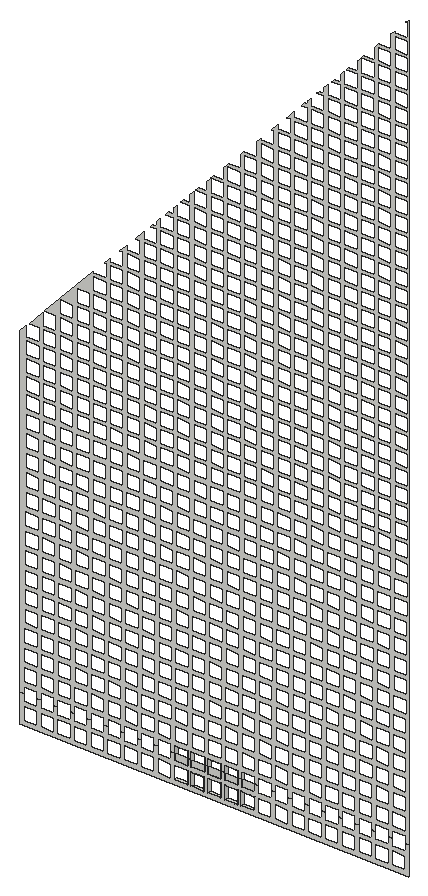
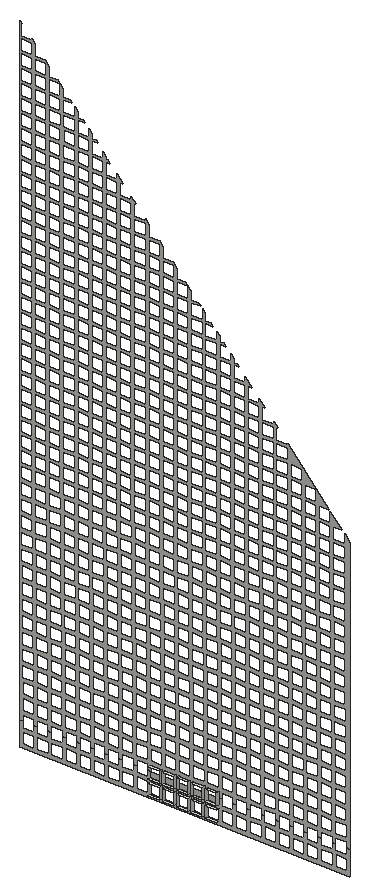
# SketchUp Ruby script. Lengths in inches.
U = 1.inch
M = Sketchup.active_model
def pt(a) = Geom::Point3d.new(a.map { |v| v * U })
def face(e, loops, mat)
  f = e.add_face(loops[0].map { |a| pt(a) })
  loops[1..].each { |l| e.add_face(l.map { |a| pt(a) }).erase! }
  f.material = f.back_material = mat if mat
  f
end
# faces: each face lists its corners as indices into pts; further lists are holes
def faces(e, pts, list, mat = nil) = list.each { |f| face(e, (f[0].is_a?(Array) ? f : [f]).map { |l| l.map { |i| pts[i] } }, mat) }
# xy, xz, yz: faces in a plane at the given z, y or x. An outline is a flat list of corners, or four numbers for a rectangle; further outlines are holes
def ring(l) = l.size == 4 ? [[l[0], l[1]], [l[2], l[1]], [l[2], l[3]], [l[0], l[3]]] : l.each_slice(2).to_a
def flat(e, list, mat, &to3) = list.each { |f| face(e, (f[0].is_a?(Array) ? f : [f]).map { |l| ring(l).map { |u, v| to3.(u, v) } }, mat) }
def xy(e, z, list, mat = nil) = flat(e, list, mat) { |x, y| [x, y, z] }
def xz(e, y, list, mat = nil) = flat(e, list, mat) { |x, z| [x, y, z] }
def yz(e, x, list, mat = nil) = flat(e, list, mat) { |y, z| [x, y, z] }
def lines(e, pts, list) = list.each { |a, b| e.add_line(pt(pts[a]), pt(pts[b])) }
# prism: a flat outline (further loops are holes) pulled along v
def prism(e, loops, v, mat = nil)
  f = face(e, loops, mat); d = Geom::Vector3d.new(v.map { |x| x * U })
  f.pushpull(f.normal.samedirection?(d) ? d.length : -d.length)
end
def box(e, o, s, mat = nil) = prism(e, [[o, [o[0] + s[0], o[1], o[2]], [o[0] + s[0], o[1] + s[1], o[2]], [o[0], o[1] + s[1], o[2]]]], [0, 0, s[2]], mat)
def at(x, y, z, deg = 0) = Geom::Transformation.translation(pt([x, y, z])) * Geom::Transformation.rotation(ORIGIN, Z_AXIS, deg.degrees)
def axes(o, x, y, z) = Geom::Transformation.new([*x, 0, *y, 0, *z, 0, *pt(o).to_a, 1])
def part(name) = M.definitions.add(name)
# library, detail: a bought-in or finely detailed component or shape, given as its bounding box
def library(name, o, s) = part(name).tap { |d| box(d.entities, o, s) }
def detail(e, o, s) = box(e.add_group.entities, o, s)
def put(e, d, t, mat = nil) = e.add_instance(d, t).tap { |i| i.material = mat if mat }
def group(e, t, mat = nil) = e.add_group.tap { |g| g.transformation = t; g.material = mat if mat }.entities
root = M.entities
xy(root,259.68,[[2231.87,480.14,2234.18,480.77],[2234.78,480.14,2237.09,480.77],[2237.69,480.14,2240.01,480.77],[2240.61,480.14,2242.92,480.77],[2243.52,480.14,2245.83,480.77]])
xy(root,262,[[2231.87,480.14,2234.18,480.77],[2234.78,480.14,2237.09,480.77],[2237.69,480.14,2240.01,480.77],[2240.61,480.14,2242.92,480.77],[2243.52,480.14,2245.83,480.77]])
xy(root,262.73,[[2231.9,480.14,2234.21,480.77],[2234.8125,480.14,2237.125,480.77],[2237.72,480.14,2240.04,480.77],[2240.64,480.14,2242.95,480.77],[2243.55,480.14,2245.86,480.77]])
xy(root,265.04,[[2231.9,480.14,2234.21,480.77],[2234.8125,480.14,2237.125,480.77],[2237.72,480.14,2240.04,480.77],[2240.64,480.14,2242.95,480.77],[2243.55,480.14,2245.86,480.77]])
xz(root,480.14,[[[2205.04,258.95,2272.64,258.95,2272.64,263.89,2272.07,263.89,2272.07,262.73,2269.76,262.73,2269.76,263.89,2269.16,263.89,2269.16,262.73,2266.84,262.73,2266.84,263.89,2266.24,263.89,2266.24,262.73,2263.93,262.73,2263.93,263.89,2263.33,263.89,2263.33,262.73,2261.02,262.73,2261.02,263.89,2260.42,263.89,2260.42,262.73,2258.11,262.73,2258.11,263.89,2257.51,263.89,2257.51,262.73,2255.2,262.73,2255.2,263.89,2254.6,263.89,2254.6,262.73,2252.28,262.73,2252.28,263.89,2251.68,263.89,2251.68,262.73,2249.37,262.73,2249.37,263.89,2248.77,263.89,2248.77,262.73,2246.46,262.73,2246.46,263.89,2245.86,263.89,2245.86,262.73,2243.55,262.73,2243.55,263.89,2242.95,263.89,2242.95,262.73,2240.64,262.73,2240.64,263.89,2240.04,263.89,2240.04,262.73,2237.72,262.73,2237.72,263.89,2237.125,263.89,2237.125,262.73,2234.8125,262.73,2234.8125,263.89,2234.21,263.89,2234.21,262.73,2231.9,262.73,2231.9,263.89,2231.3,263.89,2231.3,262.73,2228.99,262.73,2228.99,263.89,2228.39,263.89,2228.39,262.73,2226.08,262.73,2226.08,263.89,2225.48,263.89,2225.48,262.73,2223.16,262.73,2223.16,263.89,2222.5625,263.89,2222.5625,262.73,2220.25,262.73,2220.25,263.89,2219.65,263.89,2219.65,262.73,2217.34,262.73,2217.34,263.89,2216.74,263.89,2216.74,262.73,2214.43,262.73,2214.43,263.89,2213.83,263.89,2213.83,262.73,2211.52,262.73,2211.52,263.89,2210.92,263.89,2210.92,262.73,2208.6,262.73,2208.6,263.89,2208,263.89,2208,262.73,2205.69,262.73,2205.69,263.89,2205.04,263.89],[2269.73,259.68,2272.04,262],[2266.81,259.68,2269.13,262],[2263.9,259.68,2266.22,262],[2260.99,259.68,2263.3,262],[2258.08,259.68,2260.39,262],[2255.17,259.68,2257.48,262],[2252.25,259.68,2254.57,262],[2249.34,259.68,2251.66,262],[2246.43,259.68,2248.74,262],[2243.52,259.68,2245.83,262],[2240.61,259.68,2242.92,262],[2237.69,259.68,2240.01,262],[2234.78,259.68,2237.09,262],[2231.87,259.68,2234.18,262],[2228.96,259.68,2231.27,262],[2226.05,259.68,2228.36,262],[2223.13,259.68,2225.45,262],[2220.22,259.68,2222.53,262],[2217.31,259.68,2219.62,262],[2214.4,259.68,2216.71,262],[2211.49,259.68,2213.8,262],[2208.57,259.68,2210.89,262],[2205.66,259.68,2207.97,262]],[2231.9,262.73,2234.21,263.89],[2234.8125,262.73,2237.125,263.89],[2237.72,262.73,2240.04,263.89],[2240.64,262.73,2242.95,263.89],
  [2243.55,262.73,2245.86,263.89],[[2205.04,263.89,2205.69,263.89,2205.69,265.04,2208,265.04,2208,263.89,2208.6,263.89,2208.6,265.04,2210.92,265.04,2210.92,263.89,2211.52,263.89,2211.52,265.04,2213.83,265.04,2213.83,263.89,2214.43,263.89,2214.43,265.04,2216.74,265.04,2216.74,263.89,2217.34,263.89,2217.34,265.04,2219.65,265.04,2219.65,263.89,2220.25,263.89,2220.25,265.04,2222.5625,265.04,2222.5625,263.89,2223.16,263.89,2223.16,265.04,2225.48,265.04,2225.48,263.89,2226.08,263.89,2226.08,265.04,2228.39,265.04,2228.39,263.89,2228.99,263.89,2228.99,265.04,2231.3,265.04,2231.3,263.89,2231.9,263.89,2231.9,265.04,2234.21,265.04,2234.21,263.89,2234.8125,263.89,2234.8125,265.04,2237.125,265.04,2237.125,263.89,2237.72,263.89,2237.72,265.04,2240.04,265.04,2240.04,263.89,2240.64,263.89,2240.64,265.04,2242.95,265.04,2242.95,263.89,2243.55,263.89,2243.55,265.04,2245.86,265.04,2245.86,263.89,2246.46,263.89,2246.46,265.04,2248.77,265.04,2248.77,263.89,2249.37,263.89,2249.37,265.04,2251.68,265.04,2251.68,263.89,2252.28,263.89,2252.28,265.04,2254.6,265.04,2254.6,263.89,2255.2,263.89,2255.2,265.04,2257.51,265.04,2257.51,263.89,2258.11,263.89,2258.11,265.04,2260.42,265.04,2260.42,263.89,2261.02,263.89,2261.02,265.04,2263.33,265.04,2263.33,263.89,2263.93,263.89,2263.93,265.04,2266.24,265.04,2266.24,263.89,2266.84,263.89,2266.84,265.04,2269.16,265.04,2269.16,263.89,2269.76,263.89,2269.76,265.04,2272.07,265.04,2272.07,263.89,2272.64,263.89,2272.64,392.36,2272.21,391.9,2272.5,391.9,2272.5,389.59,2270.19,389.59,2270.19,389.75,2269.59,389.11,2269.59,386.84,2267.46,386.84,2266.68,386,2266.68,384.09,2264.89,384.09,2264.57,383.75,2264.48,383.65,2266.68,383.65,2266.68,381.34,2264.37,381.34,2264.37,383.53,2263.77,382.89,2263.77,381.34,2262.31,381.34,2261.9,380.9,2263.77,380.9,2263.77,378.59,2261.45,378.59,2261.45,380.43,2260.86,379.79,2260.86,378.59,2259.73,378.59,2259.32,378.15,2260.86,378.15,2260.86,375.84,2258.54,375.84,2258.54,377.32,2257.94,376.68,2257.94,375.84,2257.15,375.84,2256.74,375.4,2257.94,375.4,2257.94,373.09,2255.63,373.09,2255.63,374.21,2255.03,373.57,2255.03,373.09,2254.58,373.09,2254.11,372.59,2255.03,372.59,2255.03,370.27,2252.72,370.27,2252.72,371.11,2252.12,370.47,2252.12,370.27,2251.94,370.27,2251.47,369.77,2252.12,369.77,2252.12,367.46,2249.81,367.46,2249.81,368,2248.83,366.96,2249.21,366.96,2249.21,364.65,2246.89,364.65,2246.89,364.89,2246.2,364.15,2246.29,364.15,2246.29,361.84,2244.03,361.84,2243.38,361.14,2243.38,359.02,2241.4,359.02,2240.47,358.04,2240.47,356.21,2238.76,356.21,2238.29,355.71,2240.47,355.71,2240.47,353.4,2238.16,353.4,2238.16,355.57,2237.56,354.93,2237.56,353.4,2236.12,353.4,2235.65,352.9,2237.56,352.9,2237.56,350.59,2235.25,350.59,2235.25,352.46,2234.65,351.82,2234.65,350.59,2233.49,350.59,2233.02,350.09,2234.65,350.09,2234.65,347.77,2232.33,347.77,2232.33,349.36,2231.73,348.72,2231.73,347.77,2230.85,347.77,2230.38,347.27,2231.73,347.27,2231.73,344.96,2229.42,344.96,2229.42,346.25,2228.82,345.61,2228.82,344.96,2228.21,344.96,2227.75,344.46,2228.82,344.46,2228.82,342.15,2226.51,342.15,2226.51,343.14,2225.11,341.65,2225.91,341.65,2225.91,339.34,2223.6,339.34,2223.6,340.04,2222.47,338.84,2223,338.84,2223,336.52,2220.6875,336.52,2220.6875,336.93,2219.84,336.02,2220.09,336.02,2220.09,333.71,2217.77,333.71,2217.77,333.82,2209.29,324.77,2211.35,324.77,2211.35,322.46,2209.04,322.46,2209.04,324.5,2206.66,321.96,2208.4375,321.96,2208.4375,319.65,2206.125,319.65,2206.125,321.39,2205.04,320.24],[2270.19,375.84,2272.5,378.15],[2267.25,373.09,2269.57,375.4],[2270.19,373.09,2272.5,375.4],[2267.25,370.27,2269.57,372.59],[2270.19,370.27,2272.5,372.59],[2258.52,370.27,2260.83,372.59],[2261.45,370.27,2263.77,372.59],[2261.43,373.09,2263.74,375.4],[2264.37,373.09,2266.68,375.4],[2264.34,375.84,2266.65,378.15],[2267.28,375.84,2269.59,378.15],[2267.25,378.59,2269.57,380.9],[2270.19,378.59,2272.5,380.9],[2267.25,381.34,2269.57,383.65],[2270.19,381.34,2272.5,383.65],[2238.16,350.59,2240.47,352.9],[2235.25,347.77,2237.56,350.09],[2238.16,347.77,2240.47,350.09],[2232.33,344.96,2234.65,347.27],[2235.25,344.96,2237.56,347.27],[2238.16,344.96,2240.47,347.27],[2241.07,344.96,2243.38,347.27],[2243.98,344.96,2246.29,347.27],[2246.89,344.96,2249.21,347.27],[2249.81,344.96,2252.12,347.27],[2252.72,344.96,2255.03,347.27],[2255.63,344.96,2257.94,347.27],[2258.54,344.96,2260.86,347.27],[2261.45,344.96,2263.77,347.27],[2264.37,344.96,2266.68,347.27],[2267.28,344.96,2269.59,347.27],[2270.19,344.96,2272.5,347.27],[2241.07,347.77,2243.38,350.09],[2243.98,347.77,2246.29,350.09],[2246.89,347.77,2249.21,350.09],[2249.81,347.77,2252.12,350.09],[2252.72,347.77,2255.03,350.09],[2255.63,347.77,2257.94,350.09],[2258.54,347.77,2260.86,350.09],[2261.45,347.77,2263.77,350.09],[2264.37,347.77,2266.68,350.09],[2267.28,347.77,2269.59,350.09],[2270.19,347.77,2272.5,350.09],[2241.07,350.59,2243.38,352.9],[2243.98,350.59,2246.29,352.9],[2246.89,350.59,2249.21,352.9],[2249.81,350.59,2252.12,352.9],[2252.72,350.59,2255.03,352.9],[2255.63,350.59,2257.94,352.9],[2258.54,350.59,2260.86,352.9],[2261.45,350.59,2263.77,352.9],[2264.37,350.59,2266.68,352.9],[2267.28,350.59,2269.59,352.9],[2270.19,350.59,2272.5,352.9],[2241.07,353.4,2243.38,355.71],[2243.98,353.4,2246.29,355.71],[2246.89,353.4,2249.21,355.71],[2249.81,353.4,2252.12,355.71],[2252.72,353.4,2255.03,355.71],[2255.63,353.4,2257.94,355.71],[2258.54,353.4,2260.86,355.71],[2261.45,353.4,2263.77,355.71],[2264.37,353.4,2266.68,355.71],[2267.28,353.4,2269.59,355.71],[2270.19,353.4,2272.5,355.71],[2252.72,367.46,2255.03,369.77],[2255.63,367.46,2257.94,369.77],[2264.37,367.46,2266.68,369.77],[2270.19,367.46,2272.5,369.77],[2261.45,367.46,2263.77,369.77],[2258.54,367.46,2260.86,369.77],[2267.28,367.46,2269.59,369.77],[2252.72,364.65,2255.03,366.96],[2258.54,364.65,2260.86,366.96],[2267.28,364.65,2269.59,366.96],[2264.37,364.65,2266.68,366.96],[2255.63,364.65,2257.94,366.96],[2261.45,364.65,2263.77,366.96],[2270.19,364.65,2272.5,366.96],[2249.81,364.65,2252.12,366.96],[2261.45,361.84,2263.77,364.15],[2267.28,361.84,2269.59,364.15],[2255.63,361.84,2257.94,364.15],[2258.54,361.84,2260.86,364.15],[2270.19,361.84,2272.5,364.15],[2249.81,361.84,2252.12,364.15],[2246.89,361.84,2249.21,364.15],[2252.72,361.84,2255.03,364.15],[2264.37,361.84,2266.68,364.15],[2261.45,359.02,2263.77,361.34],[2267.28,359.02,2269.59,361.34],[2255.63,359.02,2257.94,361.34],[2243.98,359.02,2246.29,361.34],[2270.19,359.02,2272.5,361.34],[2258.54,359.02,2260.86,361.34],[2249.81,359.02,2252.12,361.34],[2246.89,359.02,2249.21,361.34],[2264.37,359.02,2266.68,361.34],[2252.72,359.02,2255.03,361.34],[2264.37,356.21,2266.68,358.52],[2252.72,356.21,2255.03,358.52],[2246.89,356.21,2249.21,358.52],[2258.54,356.21,2260.86,358.52],[2270.19,356.21,2272.5,358.52],[2241.07,356.21,2243.38,358.52],[2249.81,356.21,2252.12,358.52],[2243.98,356.21,2246.29,358.52],[2255.63,356.21,2257.94,358.52],[2267.28,356.21,2269.59,358.52],[2261.45,356.21,2263.77,358.52],[2229.42,342.15,2231.73,344.46],[2232.33,342.15,2234.65,344.46],[2235.25,342.15,2237.56,344.46],[2238.16,342.15,2240.47,344.46],[2241.07,342.15,2243.38,344.46],[2243.98,342.15,2246.29,344.46],[2246.89,342.15,2249.21,344.46],[2249.81,342.15,2252.12,344.46],[2252.72,342.15,2255.03,344.46],[2255.63,342.15,2257.94,344.46],[2258.54,342.15,2260.86,344.46],[2261.45,342.15,2263.77,344.46],[2264.37,342.15,2266.68,344.46],[2267.28,342.15,2269.59,344.46],[2270.19,342.15,2272.5,344.46],[2226.51,339.34,2228.82,341.65],[2229.42,339.34,2231.73,341.65],[2232.33,339.34,2234.65,341.65],[2235.25,339.34,2237.56,341.65],[2238.16,339.34,2240.47,341.65],[2241.07,339.34,2243.38,341.65],[2243.98,339.34,2246.29,341.65],[2246.89,339.34,2249.21,341.65],[2249.81,339.34,2252.12,341.65],[2252.72,339.34,2255.03,341.65],[2255.63,339.34,2257.94,341.65],[2258.54,339.34,2260.86,341.65],[2261.45,339.34,2263.77,341.65],[2264.37,339.34,2266.68,341.65],[2267.28,339.34,2269.59,341.65],[2270.19,339.34,2272.5,341.65],[2223.6,336.52,2225.91,338.84],[2226.51,336.52,2228.82,338.84],[2229.42,336.52,2231.73,338.84],[2232.33,336.52,2234.65,338.84],[2235.25,336.52,2237.56,338.84],[2238.16,336.52,2240.47,338.84],[2241.07,336.52,2243.38,338.84],[2243.98,336.52,2246.29,338.84],[2246.89,336.52,2249.21,338.84],[2249.81,336.52,2252.12,338.84],[2252.72,336.52,2255.03,338.84],[2255.63,336.52,2257.94,338.84],[2258.54,336.52,2260.86,338.84],[2261.45,336.52,2263.77,338.84],[2264.37,336.52,2266.68,338.84],[2267.28,336.52,2269.59,338.84],[2270.19,336.52,2272.5,338.84],[2220.6875,333.71,2223,336.02],[2223.6,333.71,2225.91,336.02],[2226.51,333.71,2228.82,336.02],[2229.42,333.71,2231.73,336.02],[2232.33,333.71,2234.65,336.02],[2235.25,333.71,2237.56,336.02],[2238.16,333.71,2240.47,336.02],[2241.07,333.71,2243.38,336.02],[2243.98,333.71,2246.29,336.02],[2246.89,333.71,2249.21,336.02],[2249.81,333.71,2252.12,336.02],[2252.72,333.71,2255.03,336.02],[2255.63,333.71,2257.94,336.02],[2258.54,333.71,2260.86,336.02],[2261.45,333.71,2263.77,336.02],[2264.37,333.71,2266.68,336.02],[2267.28,333.71,2269.59,336.02],[2270.19,333.71,2272.5,336.02],[2217.77,330.9,2220.09,333.21],[2220.6875,330.9,2223,333.21],[2223.6,330.9,2225.91,333.21],[2226.51,330.9,2228.82,333.21],[2229.42,330.9,2231.73,333.21],[2232.33,330.9,2234.65,333.21],[2235.25,330.9,2237.56,333.21],[2238.16,330.9,2240.47,333.21],[2241.07,330.9,2243.38,333.21],[2243.98,330.9,2246.29,333.21],[2246.89,330.9,2249.21,333.21],[2249.81,330.9,2252.12,333.21],[2252.72,330.9,2255.03,333.21],[2255.63,330.9,2257.94,333.21],[2258.54,330.9,2260.86,333.21],[2261.45,330.9,2263.77,333.21],[2264.37,330.9,2266.68,333.21],[2267.28,330.9,2269.59,333.21],[2270.19,330.9,2272.5,333.21],[2214.86,328.09,2217.17,330.4],[2217.77,328.09,2220.09,330.4],[2220.6875,328.09,2223,330.4],[2223.6,328.09,2225.91,330.4],[2226.51,328.09,2228.82,330.4],[2229.42,328.09,2231.73,330.4],[2232.33,328.09,2234.65,330.4],[2235.25,328.09,2237.56,330.4],[2238.16,328.09,2240.47,330.4],[2241.07,328.09,2243.38,330.4],[2243.98,328.09,2246.29,330.4],[2246.89,328.09,2249.21,330.4],[2249.81,328.09,2252.12,330.4],[2252.72,328.09,2255.03,330.4],[2255.63,328.09,2257.94,330.4],[2258.54,328.09,2260.86,330.4],[2261.45,328.09,2263.77,330.4],[2264.37,328.09,2266.68,330.4],[2267.28,328.09,2269.59,330.4],[2270.19,328.09,2272.5,330.4],[2211.95,325.27,2214.26,327.59],[2214.86,325.27,2217.17,327.59],[2217.77,325.27,2220.09,327.59],[2220.6875,325.27,2223,327.59],[2223.6,325.27,2225.91,327.59],[2226.51,325.27,2228.82,327.59],[2229.42,325.27,2231.73,327.59],[2232.33,325.27,2234.65,327.59],[2235.25,325.27,2237.56,327.59],[2238.16,325.27,2240.47,327.59],[2241.07,325.27,2243.38,327.59],[2243.98,325.27,2246.29,327.59],[2246.89,325.27,2249.21,327.59],[2249.81,325.27,2252.12,327.59],[2252.72,325.27,2255.03,327.59],[2255.63,325.27,2257.94,327.59],[2258.54,325.27,2260.86,327.59],[2261.45,325.27,2263.77,327.59],[2264.37,325.27,2266.68,327.59],[2267.28,325.27,2269.59,327.59],[2270.19,325.27,2272.5,327.59],[2211.95,322.46,2214.26,324.77],[2214.86,322.46,2217.17,324.77],[2217.77,322.46,2220.09,324.77],[2220.6875,322.46,2223,324.77],[2223.6,322.46,2225.91,324.77],[2226.51,322.46,2228.82,324.77],[2229.42,322.46,2231.73,324.77],[2232.33,322.46,2234.65,324.77],[2235.25,322.46,2237.56,324.77],[2238.16,322.46,2240.47,324.77],[2241.07,322.46,2243.38,324.77],[2243.98,322.46,2246.29,324.77],[2246.89,322.46,2249.21,324.77],[2249.81,322.46,2252.12,324.77],[2252.72,322.46,2255.03,324.77],[2255.63,322.46,2257.94,324.77],[2258.54,322.46,2260.86,324.77],[2261.45,322.46,2263.77,324.77],[2264.37,322.46,2266.68,324.77],[2267.28,322.46,2269.59,324.77],[2270.19,322.46,2272.5,324.77],[2209.04,319.65,2211.35,321.96],[2211.95,319.65,2214.26,321.96],[2214.86,319.65,2217.17,321.96],[2217.77,319.65,2220.09,321.96],[2220.6875,319.65,2223,321.96],[2223.6,319.65,2225.91,321.96],[2226.51,319.65,2228.82,321.96],[2229.42,319.65,2231.73,321.96],[2232.33,319.65,2234.65,321.96],[2235.25,319.65,2237.56,321.96],[2238.16,319.65,2240.47,321.96],[2241.07,319.65,2243.38,321.96],[2243.98,319.65,2246.29,321.96],[2246.89,319.65,2249.21,321.96],[2249.81,319.65,2252.12,321.96],[2252.72,319.65,2255.03,321.96],[2255.63,319.65,2257.94,321.96],[2258.54,319.65,2260.86,321.96],[2261.45,319.65,2263.77,321.96],[2264.37,319.65,2266.68,321.96],[2267.28,319.65,2269.59,321.96],[2270.19,319.65,2272.5,321.96],[2206.125,316.84,2208.4375,319.15],[2209.04,316.84,2211.35,319.15],[2211.95,316.84,2214.26,319.15],[2214.86,316.84,2217.17,319.15],[2217.77,316.84,2220.09,319.15],[2220.6875,316.84,2223,319.15],[2223.6,316.84,2225.91,319.15],[2226.51,316.84,2228.82,319.15],[2229.42,316.84,2231.73,319.15],[2232.33,316.84,2234.65,319.15],[2235.25,316.84,2237.56,319.15],[2238.16,316.84,2240.47,319.15],[2241.07,316.84,2243.38,319.15],[2243.98,316.84,2246.29,319.15],[2246.89,316.84,2249.21,319.15],[2249.81,316.84,2252.12,319.15],[2252.72,316.84,2255.03,319.15],[2255.63,316.84,2257.94,319.15],[2258.54,316.84,2260.86,319.15],[2261.45,316.84,2263.77,319.15],[2264.37,316.84,2266.68,319.15],[2267.28,316.84,2269.59,319.15],[2270.19,316.84,2272.5,319.15],[2206.125,314.02,2208.4375,316.34],[2209.04,314.02,2211.35,316.34],[2211.95,314.02,2214.26,316.34],[2214.86,314.02,2217.17,316.34],[2217.77,314.02,2220.09,316.34],[2220.6875,314.02,2223,316.34],[2223.6,314.02,2225.91,316.34],[2226.51,314.02,2228.82,316.34],[2229.42,314.02,2231.73,316.34],[2232.33,314.02,2234.65,316.34],[2235.25,314.02,2237.56,316.34],[2238.16,314.02,2240.47,316.34],[2241.07,314.02,2243.38,316.34],[2243.98,314.02,2246.29,316.34],[2246.89,314.02,2249.21,316.34],[2249.81,314.02,2252.12,316.34],[2252.72,314.02,2255.03,316.34],[2255.63,314.02,2257.94,316.34],[2258.54,314.02,2260.86,316.34],[2261.45,314.02,2263.77,316.34],[2264.37,314.02,2266.68,316.34],[2267.28,314.02,2269.59,316.34],[2270.19,314.02,2272.5,316.34],[2223.6,311.21,2225.91,313.52],[2226.51,311.21,2228.82,313.52],[2211.95,311.21,2214.26,313.52],[2206.125,311.21,2208.4375,313.52],[2267.28,311.21,2269.59,313.52],[2249.81,311.21,2252.12,313.52],[2238.16,311.21,2240.47,313.52],[2214.86,311.21,2217.17,313.52],[2243.98,311.21,2246.29,313.52],[2241.07,311.21,2243.38,313.52],[2217.77,311.21,2220.09,313.52],[2255.63,311.21,2257.94,313.52],[2229.42,311.21,2231.73,313.52],[2264.37,311.21,2266.68,313.52],[2258.54,311.21,2260.86,313.52],[2209.04,311.21,2211.35,313.52],[2252.72,311.21,2255.03,313.52],[2261.45,311.21,2263.77,313.52],[2235.25,311.21,2237.56,313.52],[2270.19,311.21,2272.5,313.52],[2220.6875,311.21,2223,313.52],[2232.33,311.21,2234.65,313.52],[2246.89,311.21,2249.21,313.52],[2206.125,308.4,2208.4375,310.71],[2209.04,308.4,2211.35,310.71],[2211.95,308.4,2214.26,310.71],[2214.86,308.4,2217.17,310.71],[2217.77,308.4,2220.09,310.71],[2220.6875,308.4,2223,310.71],[2223.6,308.4,2225.91,310.71],[2226.51,308.4,2228.82,310.71],[2229.42,308.4,2231.73,310.71],[2232.33,308.4,2234.65,310.71],[2235.25,308.4,2237.56,310.71],[2238.16,308.4,2240.47,310.71],[2241.07,308.4,2243.38,310.71],[2243.98,308.4,2246.29,310.71],[2246.89,308.4,2249.21,310.71],[2249.81,308.4,2252.12,310.71],[2252.72,308.4,2255.03,310.71],[2255.63,308.4,2257.94,310.71],[2258.54,308.4,2260.86,310.71],[2261.45,308.4,2263.77,310.71],[2264.37,308.4,2266.68,310.71],[2267.28,308.4,2269.59,310.71],[2270.19,308.4,2272.5,310.71],[2206.1,305.35,2208.41,307.67],[2209.01,305.35,2211.32,307.67],[2211.92,305.35,2214.23,307.67],[2214.83,305.35,2217.15,307.67],[2217.75,305.35,2220.06,307.67],[2220.66,305.35,2222.97,307.67],[2223.57,305.35,2225.88,307.67],[2226.48,305.35,2228.79,307.67],[2229.39,305.35,2231.71,307.67],[2232.31,305.35,2234.62,307.67],[2235.22,305.35,2237.53,307.67],[2238.13,305.35,2240.44,307.67],[2241.04,305.35,2243.35,307.67],[2243.95,305.35,2246.27,307.67],[2246.87,305.35,2249.18,307.67],[2249.78,305.35,2252.09,307.67],[2252.6875,305.35,2255,307.67],[2255.6,305.35,2257.91,307.67],[2258.51,305.35,2260.83,307.67],[2261.43,305.35,2263.74,307.67],[2264.34,305.35,2266.65,307.67],[2267.25,305.35,2269.5625,307.67],[2270.16,305.35,2272.47,307.67],[2206.07,302.31,2208.38,304.62],[2208.98,302.31,2211.29,304.62],[2211.89,302.31,2214.2,304.62],[2214.8,302.31,2217.12,304.62],[2217.72,302.31,2220.03,304.62],[2220.63,302.31,2222.94,304.62],[2223.54,302.31,2225.85,304.62],[2226.45,302.31,2228.76,304.62],[2229.36,302.31,2231.68,304.62],[2232.28,302.31,2234.59,304.62],[2235.1875,302.31,2237.5,304.62],[2238.1,302.31,2240.41,304.62],[2241.01,302.31,2243.32,304.62],[2243.92,302.31,2246.24,304.62],[2246.84,302.31,2249.15,304.62],[2249.75,302.31,2252.0625,304.62],[2252.66,302.31,2254.97,304.62],[2255.57,302.31,2257.89,304.62],[2258.48,302.31,2260.8,304.62],[2261.4,302.31,2263.71,304.62],[2264.31,302.31,2266.62,304.62],[2267.22,302.31,2269.53,304.62],[2270.13,302.31,2272.45,304.62],[2206.04,299.27,2208.35,301.58],[2208.95,299.27,2211.26,301.58],[2211.86,299.27,2214.18,301.58],[2214.78,299.27,2217.09,301.58],[2217.6875,299.27,2220,301.58],[2220.6,299.27,2222.91,301.58],[2223.51,299.27,2225.82,301.58],[2226.42,299.27,2228.74,301.58],[2229.34,299.27,2231.65,301.58],[2232.25,299.27,2234.56,301.58],[2235.16,299.27,2237.47,301.58],[2238.07,299.27,2240.38,301.58],[2240.98,299.27,2243.3,301.58],[2243.9,299.27,2246.21,301.58],[2246.81,299.27,2249.12,301.58],[2249.72,299.27,2252.03,301.58],[2252.63,299.27,2254.94,301.58],[2255.54,299.27,2257.86,301.58],[2258.46,299.27,2260.77,301.58],[2261.37,299.27,2263.68,301.58],[2264.28,299.27,2266.59,301.58],[2267.19,299.27,2269.5,301.58],[2270.1,299.27,2272.42,301.58],[2206.01,296.22,2208.32,298.53],[2208.92,296.22,2211.23,298.53],[2211.83,296.22,2214.15,298.53],[2214.75,296.22,2217.06,298.53],[2217.66,296.22,2219.97,298.53],[2220.57,296.22,2222.88,298.53],[2223.48,296.22,2225.79,298.53],[2226.39,296.22,2228.71,298.53],[2229.31,296.22,2231.62,298.53],[2232.22,296.22,2234.53,298.53],[2235.13,296.22,2237.44,298.53],[2238.04,296.22,2240.35,298.53],[2240.95,296.22,2243.27,298.53],[2243.87,296.22,2246.18,298.53],[2246.78,296.22,2249.09,298.53],[2249.69,296.22,2252,298.53],[2252.6,296.22,2254.91,298.53],[2255.51,296.22,2257.83,298.53],[2258.43,296.22,2260.74,298.53],[2261.34,296.22,2263.65,298.53],[2264.25,296.22,2266.5625,298.53],[2267.16,296.22,2269.48,298.53],[2270.07,296.22,2272.39,298.53],[2205.98,293.18,2208.29,295.49],[2208.89,293.18,2211.21,295.49],[2211.8,293.18,2214.12,295.49],[2214.72,293.18,2217.03,295.49],[2217.63,293.18,2219.94,295.49],[2220.54,293.18,2222.85,295.49],[2223.45,293.18,2225.77,295.49],[2226.37,293.18,2228.68,295.49],[2229.28,293.18,2231.59,295.49],[2232.1875,293.18,2234.5,295.49],[2235.1,293.18,2237.41,295.49],[2238.01,293.18,2240.33,295.49],[2240.93,293.18,2243.24,295.49],[2243.84,293.18,2246.15,295.49],[2246.75,293.18,2249.0625,295.49],[2249.66,293.18,2251.97,295.49],[2252.57,293.18,2254.89,295.49],[2255.49,293.18,2257.8,295.49],[2258.4,293.18,2260.71,295.49],[2261.31,293.18,2263.62,295.49],[2264.22,293.18,2266.53,295.49],[2267.13,293.18,2269.45,295.49],[2270.05,293.18,2272.36,295.49],[2205.95,290.13,2208.26,292.44],[2208.86,290.13,2211.18,292.44],[2211.78,290.13,2214.09,292.44],[2214.6875,290.13,2217,292.44],[2217.6,290.13,2219.91,292.44],[2220.51,290.13,2222.82,292.44],[2223.42,290.13,2225.74,292.44],[2226.34,290.13,2228.65,292.44],[2229.25,290.13,2231.5625,292.44],[2232.16,290.13,2234.47,292.44],[2235.07,290.13,2237.38,292.44],[2237.98,290.13,2240.3,292.44],[2240.9,290.13,2243.21,292.44],[2243.81,290.13,2246.12,292.44],[2246.72,290.13,2249.03,292.44],[2249.63,290.13,2251.94,292.44],[2252.54,290.13,2254.86,292.44],[2255.46,290.13,2257.77,292.44],[2258.37,290.13,2260.68,292.44],[2261.28,290.13,2263.59,292.44],[2264.19,290.13,2266.51,292.44],[2267.1,290.13,2269.42,292.44],[2270.02,290.13,2272.33,292.44],[2205.92,287.09,2208.24,289.4],[2208.83,287.09,2211.15,289.4],[2211.75,287.09,2214.06,289.4],[2214.66,287.09,2216.97,289.4],[2217.57,287.09,2219.88,289.4],[2220.48,287.09,2222.8,289.4],[2223.4,287.09,2225.71,289.4],[2226.31,287.09,2228.62,289.4],[2229.22,287.09,2231.53,289.4],[2232.13,287.09,2234.44,289.4],[2235.04,287.09,2237.36,289.4],[2237.96,287.09,2240.27,289.4],[2240.87,287.09,2243.18,289.4],[2243.78,287.09,2246.09,289.4],[2246.69,287.09,2249,289.4],[2249.6,287.09,2251.92,289.4],[2252.52,287.09,2254.83,289.4],[2255.43,287.09,2257.74,289.4],[2258.34,287.09,2260.65,289.4],[2261.25,287.09,2263.5625,289.4],[2264.16,287.09,2266.48,289.4],[2267.08,287.09,2269.39,289.4],[2269.99,287.09,2272.3,289.4],[2205.89,284.04,2208.21,286.35],[2208.81,284.04,2211.12,286.35],[2211.72,284.04,2214.03,286.35],[2214.63,284.04,2216.94,286.35],[2217.54,284.04,2219.85,286.35],[2220.45,284.04,2222.77,286.35],[2223.37,284.04,2225.68,286.35],[2226.28,284.04,2228.59,286.35],[2229.19,284.04,2231.5,286.35],[2232.1,284.04,2234.41,286.35],[2235.01,284.04,2237.33,286.35],[2237.93,284.04,2240.24,286.35],[2240.84,284.04,2243.15,286.35],[2243.75,284.04,2246.0625,286.35],[2246.66,284.04,2248.97,286.35],[2249.57,284.04,2251.89,286.35],[2252.49,284.04,2254.8,286.35],[2255.4,284.04,2257.71,286.35],[2258.3125,284.04,2260.625,286.35],[2261.22,284.04,2263.54,286.35],[2264.13,284.04,2266.45,286.35],[2267.05,284.04,2269.36,286.35],[2269.96,284.04,2272.27,286.35],[2205.86,281,2208.18,283.31],[2208.78,281,2211.09,283.31],[2211.6875,281,2214,283.31],[2214.6,281,2216.91,283.31],[2217.51,281,2219.83,283.31],[2220.43,281,2222.74,283.31],[2223.34,281,2225.65,283.31],[2226.25,281,2228.5625,283.31],[2229.16,281,2231.47,283.31],[2232.07,281,2234.39,283.31],[2234.99,281,2237.3,283.31],[2237.9,281,2240.21,283.31],[2240.81,281,2243.12,283.31],[2243.72,281,2246.03,283.31],[2246.63,281,2248.95,283.31],[2249.55,281,2251.86,283.31],[2252.46,281,2254.77,283.31],[2255.37,281,2257.68,283.31],[2258.28,281,2260.59,283.31],[2261.19,281,2263.51,283.31],[2264.11,281,2266.42,283.31],[2267.02,281,2269.33,283.31],[2269.93,281,2272.24,283.31],[2205.84,277.95,2208.15,280.26],[2208.75,277.95,2211.06,280.26],[2211.66,277.95,2213.97,280.26],[2214.57,277.95,2216.88,280.26],[2217.48,277.95,2219.8,280.26],[2220.4,277.95,2222.71,280.26],[2223.31,277.95,2225.62,280.26],[2226.22,277.95,2228.53,280.26],[2229.13,277.95,2231.44,280.26],[2232.04,277.95,2234.36,280.26],[2234.96,277.95,2237.27,280.26],[2237.87,277.95,2240.18,280.26],[2240.78,277.95,2243.09,280.26],[2243.69,277.95,2246,280.26],[2246.6,277.95,2248.92,280.26],[2249.52,277.95,2251.83,280.26],[2252.43,277.95,2254.74,280.26],[2255.34,277.95,2257.65,280.26],[2258.25,277.95,2260.57,280.26],[2261.16,277.95,2263.48,280.26],[2264.08,277.95,2266.39,280.26],[2266.99,277.95,2269.3,280.26],[2269.9,277.95,2272.21,280.26],[2205.81,274.91,2208.12,277.22],[2208.72,274.91,2211.03,277.22],[2211.63,274.91,2213.94,277.22],[2214.54,274.91,2216.86,277.22],[2217.46,274.91,2219.77,277.22],[2220.37,274.91,2222.68,277.22],[2223.28,274.91,2225.59,277.22],[2226.19,274.91,2228.5,277.22],[2229.1,274.91,2231.42,277.22],[2232.02,274.91,2234.33,277.22],[2234.93,274.91,2237.24,277.22],[2237.84,274.91,2240.15,277.22],[2240.75,274.91,2243.0625,277.22],[2243.66,274.91,2245.98,277.22],[2246.58,274.91,2248.89,277.22],[2249.49,274.91,2251.8,277.22],[2252.4,274.91,2254.71,277.22],[2255.3125,274.91,2257.625,277.22],[2258.22,274.91,2260.54,277.22],[2261.14,274.91,2263.45,277.22],[2264.05,274.91,2266.36,277.22],[2266.96,274.91,2269.27,277.22],[2269.87,274.91,2272.18,277.22],[2205.78,271.86,2208.09,274.17],[2208.69,271.86,2211,274.17],[2211.6,271.86,2213.91,274.17],[2214.51,271.86,2216.83,274.17],[2217.43,271.86,2219.74,274.17],[2220.34,271.86,2222.65,274.17],[2223.25,271.86,2225.5625,274.17],[2226.16,271.86,2228.47,274.17],[2229.07,271.86,2231.39,274.17],[2231.99,271.86,2234.3,274.17],[2234.9,271.86,2237.21,274.17],[2237.81,271.86,2240.12,274.17],[2240.72,271.86,2243.03,274.17],[2243.63,271.86,2245.95,274.17],[2246.55,271.86,2248.86,274.17],[2249.46,271.86,2251.77,274.17],[2252.37,271.86,2254.68,274.17],[2255.28,271.86,2257.6,274.17],[2258.19,271.86,2260.51,274.17],[2261.11,271.86,2263.42,274.17],[2264.02,271.86,2266.33,274.17],[2266.93,271.86,2269.24,274.17],[2269.84,271.86,2272.16,274.17],[2205.75,268.82,2208.0625,271.13],[2208.66,268.82,2210.97,271.13],[2211.57,268.82,2213.89,271.13],[2214.49,268.82,2216.8,271.13],[2217.4,268.82,2219.71,271.13],[2220.31,268.82,2222.62,271.13],[2223.22,268.82,2225.53,271.13],[2226.13,268.82,2228.45,271.13],[2229.05,268.82,2231.36,271.13],[2231.96,268.82,2234.27,271.13],[2234.87,268.82,2237.18,271.13],[2237.78,268.82,2240.09,271.13],[2240.69,268.82,2243.01,271.13],[2243.61,268.82,2245.92,271.13],[2246.52,268.82,2248.83,271.13],[2249.43,268.82,2251.74,271.13],[2252.34,268.82,2254.65,271.13],[2255.25,268.82,2257.57,271.13],[2258.17,268.82,2260.48,271.13],[2261.08,268.82,2263.39,271.13],[2263.99,268.82,2266.3,271.13],[2266.9,268.82,2269.21,271.13],[2269.8125,268.82,2272.125,271.13],[2205.72,265.77,2208.03,268.09],[2208.63,265.77,2210.94,268.09],[2211.54,265.77,2213.86,268.09],[2214.46,265.77,2216.77,268.09],[2217.37,265.77,2219.68,268.09],[2220.28,265.77,2222.59,268.09],[2223.19,265.77,2225.5,268.09],[2226.1,265.77,2228.42,268.09],[2229.02,265.77,2231.33,268.09],[2231.93,265.77,2234.24,268.09],[2234.84,265.77,2237.15,268.09],[2237.75,265.77,2240.06,268.09],[2240.66,265.77,2242.98,268.09],[2243.58,265.77,2245.89,268.09],[2246.49,265.77,2248.8,268.09],[2249.4,265.77,2251.71,268.09],[2252.3125,265.77,2254.625,268.09],[2255.22,265.77,2257.54,268.09],[2258.14,265.77,2260.45,268.09],[2261.05,265.77,2263.36,268.09],[2263.96,265.77,2266.27,268.09],[2266.87,265.77,2269.19,268.09],[2269.78,265.77,2272.1,268.09],[2270.19,384.09,2272.5,386.4],[2267.28,384.09,2269.59,386.4],[2270.19,386.84,2272.5,389.15],[2264.37,370.27,2264.37,372.47,2264.48,372.59,2266.68,372.59,2266.68,370.27],[2255.63,370.27,2255.63,372.47,2255.74,372.59,2257.94,372.59,2257.94,370.27],[2258.54,373.09,2258.54,375.28,2258.65,375.4,2260.86,375.4,2260.86,373.09],[2261.45,375.84,2261.45,378.03,2261.5625,378.15,2263.77,378.15,2263.77,375.84],[2264.37,378.59,2264.37,380.78,2264.48,380.9,2266.68,380.9,2266.68,378.59]]])
yz(root,2231.9,[[480.14,262.73,480.77,265.04]])
yz(root,2234.18,[[480.14,259.68,480.77,262]])
yz(root,2234.21,[[480.14,262.73,480.77,265.04]])
yz(root,2234.78,[[480.14,259.68,480.77,262]])
yz(root,2234.8125,[[480.14,262.73,480.77,265.04]])
yz(root,2237.09,[[480.14,259.68,480.77,262]])
yz(root,2237.125,[[480.14,262.73,480.77,265.04]])
yz(root,2237.69,[[480.14,259.68,480.77,262]])
yz(root,2237.72,[[480.14,262.73,480.77,265.04]])
yz(root,2240.01,[[480.14,259.68,480.77,262]])
yz(root,2240.04,[[480.14,262.73,480.77,265.04]])
yz(root,2240.61,[[480.14,259.68,480.77,262]])
yz(root,2240.64,[[480.14,262.73,480.77,265.04]])
yz(root,2242.92,[[480.14,259.68,480.77,262]])
yz(root,2242.95,[[480.14,262.73,480.77,265.04]])
yz(root,2243.52,[[480.14,259.68,480.77,262]])
yz(root,2243.55,[[480.14,262.73,480.77,265.04]])
